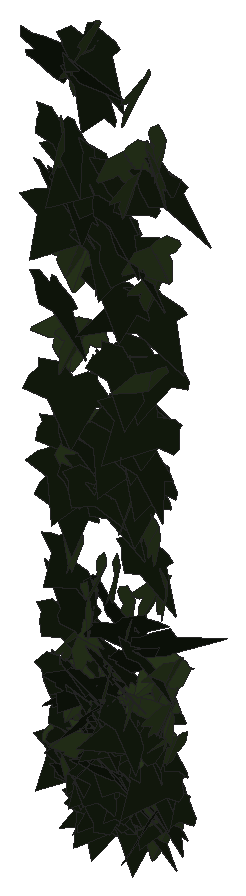
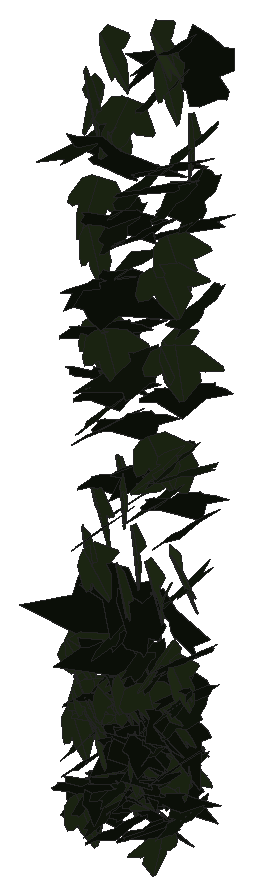
# SketchUp Ruby script. Lengths in inches.
U = 1.inch
M = Sketchup.active_model
def pt(a) = Geom::Point3d.new(a.map { |v| v * U })
def face(e, loops, mat)
  f = e.add_face(loops[0].map { |a| pt(a) })
  loops[1..].each { |l| e.add_face(l.map { |a| pt(a) }).erase! }
  f.material = f.back_material = mat if mat
  f
end
# faces: each face lists its corners as indices into pts; further lists are holes
def faces(e, pts, list, mat = nil) = list.each { |f| face(e, (f[0].is_a?(Array) ? f : [f]).map { |l| l.map { |i| pts[i] } }, mat) }
# xy, xz, yz: faces in a plane at the given z, y or x. An outline is a flat list of corners, or four numbers for a rectangle; further outlines are holes
def ring(l) = l.size == 4 ? [[l[0], l[1]], [l[2], l[1]], [l[2], l[3]], [l[0], l[3]]] : l.each_slice(2).to_a
def flat(e, list, mat, &to3) = list.each { |f| face(e, (f[0].is_a?(Array) ? f : [f]).map { |l| ring(l).map { |u, v| to3.(u, v) } }, mat) }
def xy(e, z, list, mat = nil) = flat(e, list, mat) { |x, y| [x, y, z] }
def xz(e, y, list, mat = nil) = flat(e, list, mat) { |x, z| [x, y, z] }
def yz(e, x, list, mat = nil) = flat(e, list, mat) { |y, z| [x, y, z] }
def lines(e, pts, list) = list.each { |a, b| e.add_line(pt(pts[a]), pt(pts[b])) }
# prism: a flat outline (further loops are holes) pulled along v
def prism(e, loops, v, mat = nil)
  f = face(e, loops, mat); d = Geom::Vector3d.new(v.map { |x| x * U })
  f.pushpull(f.normal.samedirection?(d) ? d.length : -d.length)
end
def box(e, o, s, mat = nil) = prism(e, [[o, [o[0] + s[0], o[1], o[2]], [o[0] + s[0], o[1] + s[1], o[2]], [o[0], o[1] + s[1], o[2]]]], [0, 0, s[2]], mat)
def at(x, y, z, deg = 0) = Geom::Transformation.translation(pt([x, y, z])) * Geom::Transformation.rotation(ORIGIN, Z_AXIS, deg.degrees)
def axes(o, x, y, z) = Geom::Transformation.new([*x, 0, *y, 0, *z, 0, *pt(o).to_a, 1])
def part(name) = M.definitions.add(name)
# library, detail: a bought-in or finely detailed component or shape, given as its bounding box
def library(name, o, s) = part(name).tap { |d| box(d.entities, o, s) }
def detail(e, o, s) = box(e.add_group.entities, o, s)
def put(e, d, t, mat = nil) = e.add_instance(d, t).tap { |i| i.material = mat if mat }
def group(e, t, mat = nil) = e.add_group.tap { |g| g.transformation = t; g.material = mat if mat }.entities
root = M.entities
M.materials.add("1026 AP 7946 SUNNY SIDE UP").color = [254, 231, 186]
M.materials.add("efeu1").color = [18, 25, 13]
M.materials.add("efeu2").color = [43, 57, 29]
c1 = part("ivyleaf_9")
p = [[1.54,2.16,1.25],[1.36,2.04,1.19],[-0.21,0.99,0.68],[-0.71,1.11,0.82],[-0.85,0.86,0.67],[-0.8,0.17,0.21],
  [-0.9,-0.01,0.1],[-0.67,-0.16,-0.02],[-0.08,-0.08,-0.05],[-0.03,-0.6,-0.4],[0.65,-0.88,-0.66],[0.83,-0.6,-0.49],
  [1.29,-0.42,-0.43],[1.8125,-0.07,-0.26],[1.21,0.44,0.15]]
faces(c1.entities,p,[[0,1,2,3,4,5,6,7,8,9,10,11,12,13,14]],"efeu1")
c2 = part("ivyleaf_10")
p = [[0,0.5,-0.03],[-0.0625,2.02,-0.43],[-0.19,2.01,-0.46],[-0.54,1.05,-0.29],[-0.52,0.625,-0.18],[-0.83,0.76,-0.28],
  [-1.16,0.64,-0.33],[-1.15,0.33,-0.24],[-0.77,-0.39,0.02],[-0.3,-0.51,0.16],[0.04,-0.48,0.23],[-0.02,2.01,-0.4375],
  [-0.06,2.01,-0.43],[0.04,-0.49,0.23],[0.67,-0.49,0.14],[1.38,0.36,-0.2],[1.375,0.51,-0.24],[0.81,0.65,-0.19],
  [0.62,0.59,-0.15],[0.6,1.09,-0.28],[0.5,1.23,-0.31]]
faces(c2.entities,p,[[0,1,2,3,4,5,6,7,8,9,10],[11,12,0,13,14,15,16,17,18,19,20]],"efeu2")
put(root,c1,axes([113.48,212.84,268.6],[-0.35522,-0.12905,0.0337],[-0.02324,-0.04117,-0.26669],[0.20833,-0.22463,0.02772]),"1026 AP 7946 SUNNY SIDE UP")
put(root,c2,axes([113.42,212.75,274.85],[-0.34565,-0.19628,0.04579],[0.03173,-0.08853,-0.29313],[0.31524,-0.2063,0.07971]),"1026 AP 7946 SUNNY SIDE UP")
put(root,c1,axes([113.22,212.86,268.37],[0.02902,-0.2292,0.12467],[0.0477,-0.11988,-0.23684],[0.40571,0.03049,0.01893]),"1026 AP 7946 SUNNY SIDE UP")
put(root,c1,axes([113.54,212.62,269.58],[-0.0128,0.25552,-0.08031],[-0.00758,-0.07957,-0.26373],[-0.42067,-0.00634,0.0072]),"1026 AP 7946 SUNNY SIDE UP")
put(root,c1,axes([113.16,212.56,277.08],[0.26409,-0.24942,0.06151],[0.02497,-0.0628,-0.30935],[0.40301,0.16733,-0.02114]),"1026 AP 7946 SUNNY SIDE UP")
put(root,c1,axes([113.01,212.5,278.9],[0.34286,-0.0936,0.22032],[0.2876,-0.11451,-0.24381],[0.22933,0.28355,-0.02363]),"1026 AP 7946 SUNNY SIDE UP")
put(root,c1,axes([113.46,212.61,276.61],[-0.26398,-0.218,0.1356],[-0.05261,-0.13886,-0.27908],[0.39797,-0.16296,0.05305]),"1026 AP 7946 SUNNY SIDE UP")
put(root,c1,axes([113.21,212.49,275.5],[0.19609,-0.27684,0.01941],[-0.00452,-0.02367,-0.31268],[0.43646,0.12413,-0.01196]),"1026 AP 7946 SUNNY SIDE UP")
put(root,c2,axes([113.47,212.67,270.32],[0.05534,-0.26982,0.04445],[0.00724,-0.04446,-0.28058],[0.42998,0.03548,-0.001]),"1026 AP 7946 SUNNY SIDE UP")
put(root,c1,axes([113.26,212.65,277.83],[0.08075,-0.29984,0.06282],[0.00263,-0.06328,-0.31363],[0.48166,0.05061,-0.00882]),"1026 AP 7946 SUNNY SIDE UP")
put(root,c1,axes([113.47,212.75,272.8125],[-0.26999,-0.22959,0.01881],[0.00256,-0.02561,-0.29501],[0.36231,-0.17091,0.0161]),"1026 AP 7946 SUNNY SIDE UP")
put(root,c1,axes([113.29,212.71,270.61],[0.05901,-0.26443,-0.07652],[0.03601,0.07622,-0.27269],[0.42975,0.02993,0.03336]),"1026 AP 7946 SUNNY SIDE UP")
put(root,c1,axes([113.35,212.71,272.41],[-0.03389,-0.28188,0.05813],[-0.00825,-0.05779,-0.29158],[0.45245,-0.02217,-0.00096]),"1026 AP 7946 SUNNY SIDE UP")
put(root,c1,axes([113.32,212.87,268.32],[0.08214,-0.25847,0.00442],[-0.01193,-0.0074,-0.27155],[0.40635,0.05203,-0.00886]),"1026 AP 7946 SUNNY SIDE UP")
put(root,c2,axes([113.35,212.77,269.06],[-0.25776,0.13858,-0.15599],[0.14481,-0.12463,-0.21982],[-0.28946,-0.18575,0.02893]),"1026 AP 7946 SUNNY SIDE UP")
put(root,c2,axes([113.53,212.86,276],[-0.28419,-0.21443,0.093],[0.0063,-0.1186,-0.27891],[0.36652,-0.16422,0.0769]),"1026 AP 7946 SUNNY SIDE UP")
put(root,c1,axes([113.32,212.83,269.125],[0.04833,-0.26355,-0.0045],[-0.00045,0.00286,-0.27333],[0.41443,0.03074,0.00023]),"1026 AP 7946 SUNNY SIDE UP")
put(root,c1,axes([113.46,212.66,271.42],[-0.1428,-0.14223,0.23774],[-0.06464,-0.23417,-0.16614],[0.42242,-0.08392,0.05495]),"1026 AP 7946 SUNNY SIDE UP")
put(root,c1,axes([113.75,212.4375,270.84],[-0.04211,0.06084,0.28221],[-0.19288,0.24457,-0.06697],[-0.39625,-0.12552,0.00261]),"1026 AP 7946 SUNNY SIDE UP")
put(root,c2,axes([113.57,212.63,276.29],[-0.12507,-0.29128,0.04301],[-0.00437,-0.04422,-0.31119],[0.46305,-0.07909,0.00868]),"1026 AP 7946 SUNNY SIDE UP")
put(root,c2,axes([113.52,212.3125,277.88],[0.16277,-0.27111,-0.13087],[0.02936,0.13842,-0.2914],[0.46884,0.08546,0.06368]),"1026 AP 7946 SUNNY SIDE UP")
put(root,c2,axes([113.55,212.8,278.88],[0.0131,-0.31323,-0.0052],[0.00308,0.00332,-0.32278],[0.49255,0.00831,0.00216]),"1026 AP 7946 SUNNY SIDE UP")
put(root,c1,axes([113.32,212.82,273.23],[-0.05087,-0.2826,0.02781],[0.15931,-0.03837,-0.27277],[0.41725,-0.0198,0.10754]),"1026 AP 7946 SUNNY SIDE UP")
put(root,c2,axes([113.54,212.56,271.76],[0.26992,-0.24753,0.01645],[-0.00644,-0.02396,-0.30997],[0.39013,0.17087,-0.01651]),"1026 AP 7946 SUNNY SIDE UP")
put(root,c2,axes([113.54,212.6875,274.89],[-0.00025,-0.25006,0.16976],[0.0574,-0.16499,-0.25665],[0.46862,0.02007,0.03153]),"1026 AP 7946 SUNNY SIDE UP")
put(root,c2,axes([113.55,212.68,269.63],[0.32708,-0.17486,-0.00281],[-0.02066,-0.01294,-0.27939],[0.27419,0.20762,-0.0177]),"1026 AP 7946 SUNNY SIDE UP")
put(root,c1,axes([113.37,212.8,269.66],[-0.04577,-0.19768,0.19034],[0.12471,-0.18499,-0.19095],[0.40804,0.03436,0.07971]),"1026 AP 7946 SUNNY SIDE UP")
put(root,c1,axes([113.375,212.54,270.01],[0.10974,-0.20238,-0.17601],[0.00466,0.17612,-0.21409],[0.41527,0.05151,0.04891]),"1026 AP 7946 SUNNY SIDE UP")
put(root,c2,axes([113.67,212.875,273.52],[-0.18295,-0.24391,0.0981],[-0.00097,-0.10543,-0.27559],[0.41251,-0.10842,0.04286]),"1026 AP 7946 SUNNY SIDE UP")
put(root,c1,axes([113.55,212.51,274.23],[-0.19164,-0.2676,-0.05532],[0.05157,0.04235,-0.30243],[0.42559,-0.12563,0.01174]),"1026 AP 7946 SUNNY SIDE UP")
put(root,c2,axes([113.63,212.8,279.27],[0.16707,-0.26335,0.1327],[0.04344,-0.129,-0.29253],[0.45996,0.10784,-0.02057]),"1026 AP 7946 SUNNY SIDE UP")
put(root,c1,axes([113.43,212.76,273.35],[0.15787,-0.27032,0.01008],[0.02044,-0.00724,-0.29694],[0.42493,0.10077,0.01054]),"1026 AP 7946 SUNNY SIDE UP")
put(root,c2,axes([113.49,212.58,273.26],[-0.02297,-0.16286,-0.29283],[0.26291,0.23995,-0.14957],[0.44151,-0.15136,0.07383]),"1026 AP 7946 SUNNY SIDE UP")
put(root,c2,axes([113.54,212.61,268.96],[0.43626,0.02874,0.04187],[0.06746,-0.02319,-0.28612],[-0.03927,0.27942,-0.02639]),"1026 AP 7946 SUNNY SIDE UP")
put(root,c1,axes([113.69,212.8,268.77],[-0.23684,-0.21018,0.04816],[-0.01429,-0.05224,-0.26566],[0.33867,-0.14918,0.02247]),"1026 AP 7946 SUNNY SIDE UP")
put(root,c2,axes([113.83,212.76,268.85],[-0.21979,-0.13195,0.18222],[-0.11105,-0.17251,-0.19028],[0.32974,-0.14605,0.05738]),"1026 AP 7946 SUNNY SIDE UP")
put(root,c1,axes([113.74,212.6875,277.39],[-0.29422,-0.1988,0.13242],[-0.04731,-0.14391,-0.27288],[0.3702,-0.17639,0.07037]),"1026 AP 7946 SUNNY SIDE UP")
put(root,c1,axes([113.53,212.625,276.97],[0.01826,-0.24914,0.18214],[0.02229,-0.17772,-0.25793],[0.48114,0.01769,0.00504]),"1026 AP 7946 SUNNY SIDE UP")
put(root,c1,axes([113.52,212.5,269.99],[0.33229,-0.15585,-0.07552],[-0.07407,0.05787,-0.26954],[0.25988,0.21577,0.01975]),"1026 AP 7946 SUNNY SIDE UP")
put(root,c2,axes([113.79,212.45,268.99],[-0.13395,-0.24571,0.08396],[-0.01971,-0.08324,-0.26797],[0.40727,-0.08484,0.01464]),"1026 AP 7946 SUNNY SIDE UP")
put(root,c1,axes([113.55,212.78,279.15],[0.1266,-0.28099,-0.12066],[-0.03861,0.11311,-0.30038],[0.47616,0.08388,0.00772]),"1026 AP 7946 SUNNY SIDE UP")
put(root,c1,axes([113.57,212.58,268.77],[-0.04031,-0.23664,0.12685],[0.07487,-0.12709,-0.23955],[0.41372,-0.00006,0.05571]),"1026 AP 7946 SUNNY SIDE UP")
put(root,c1,axes([113.56,212.73,269.77],[0.12371,-0.26151,0.00051],[0.00778,-0.00058,-0.2813],[0.41114,0.0787,0.00517]),"1026 AP 7946 SUNNY SIDE UP")
put(root,c1,axes([113.5625,212.55,272.875],[0.26404,-0.18707,-0.14183],[-0.07107,0.13902,-0.25255],[0.35724,0.16593,0.05458]),"1026 AP 7946 SUNNY SIDE UP")
put(root,c2,axes([113.8125,212.81,269.96],[-0.29711,-0.18819,0.06439],[0.01664,-0.09715,-0.26444],[0.31189,-0.17409,0.07544]),"1026 AP 7946 SUNNY SIDE UP")
put(root,c2,axes([113.72,212.71,267.83],[0.11179,0.24781,-0.00301],[-0.01534,-0.0017,-0.26545],[-0.38942,0.07121,0.00959]),"1026 AP 7946 SUNNY SIDE UP")
put(root,c1,axes([113.86,212.61,269.38],[-0.21473,0.06497,-0.22243],[0.14834,-0.21322,-0.1286],[-0.32262,-0.14128,0.08892]),"1026 AP 7946 SUNNY SIDE UP")
put(root,c1,axes([113.78,212.95,277.2],[-0.26953,-0.22433,0.0929],[-0.00009,-0.11199,-0.28378],[0.38092,-0.15876,0.06567]),"1026 AP 7946 SUNNY SIDE UP")
put(root,c1,axes([113.68,212.79,278.48],[-0.06963,-0.22261,0.21034],[-0.00907,-0.20696,-0.23353],[0.47623,-0.03649,0.0263]),"1026 AP 7946 SUNNY SIDE UP")
put(root,c2,axes([113.72,212.5,270.44],[0.06807,-0.20259,-0.22166],[0.16254,0.213,-0.18494],[0.43394,-0.04801,0.10404]),"1026 AP 7946 SUNNY SIDE UP")
put(root,c1,axes([113.95,212.35,270],[0.15929,0.17617,-0.20067],[-0.17144,-0.1629,-0.21008],[-0.37699,0.14852,0.01075]),"1026 AP 7946 SUNNY SIDE UP")
put(root,c1,axes([113.88,212.86,269.33],[-0.12185,0.11527,-0.23404],[0.1547,-0.20623,-0.14317],[-0.37049,-0.12402,0.01719]),"1026 AP 7946 SUNNY SIDE UP")
put(root,c1,axes([113.93,212.42,268.73],[-0.13152,0.18945,-0.20725],[-0.15819,0.1761,0.21381],[0.40602,0.12997,0.01617]),"1026 AP 7946 SUNNY SIDE UP")
put(root,c1,axes([113.91,212.74,267.95],[-0.19676,-0.19953,0.11969],[-0.04433,-0.11923,-0.24059],[0.36124,-0.12331,0.03567]),"1026 AP 7946 SUNNY SIDE UP")
put(root,c2,axes([113.95,212.58,271.51],[0.1304,-0.26022,-0.06907],[-0.03004,0.06272,-0.28099],[0.42089,0.0851,0.00134]),"1026 AP 7946 SUNNY SIDE UP")
put(root,c1,axes([113.69,212.375,268.59],[0.40539,0.06891,0.05745],[0.09123,-0.00307,-0.27434],[-0.10488,0.26368,-0.01656]),"1026 AP 7946 SUNNY SIDE UP")
put(root,c2,axes([113.79,212.63,271.01],[-0.00705,-0.09819,0.27508],[0.24705,-0.22413,-0.08333],[0.37393,0.14623,0.06024]),"1026 AP 7946 SUNNY SIDE UP")
put(root,c1,axes([114.07,212.85,269.23],[-0.38875,-0.10692,0.00549],[0.00653,-0.02451,-0.27652],[0.16825,-0.24609,0.02343]),"1026 AP 7946 SUNNY SIDE UP")
put(root,c2,axes([113.95,212.86,268.91],[0.03549,-0.23859,0.11226],[0.05779,-0.10678,-0.24627],[0.40927,0.03577,0.02504]),"1026 AP 7946 SUNNY SIDE UP")
put(root,c1,axes([113.93,212.73,267.97],[-0.14196,-0.23832,0.04227],[-0.01906,-0.04073,-0.26276],[0.38014,-0.09104,0.00261]),"1026 AP 7946 SUNNY SIDE UP")
put(root,c1,axes([114.33,212.68,269.55],[-0.18353,-0.01532,-0.27288],[-0.41612,-0.01263,0.12085],[-0.0279,0.2891,-0.00748]),"1026 AP 7946 SUNNY SIDE UP")
put(root,c1,axes([113.8,212.86,269.1],[0.02233,-0.22202,0.14867],[0.07158,-0.14159,-0.22786],[0.41127,0.0367,0.03159]),"1026 AP 7946 SUNNY SIDE UP")
put(root,c1,axes([114.11,212.57,269.05],[0.02433,0.26408,-0.04313],[-0.00187,-0.04336,-0.27277],[-0.4208,0.01546,-0.00128]),"1026 AP 7946 SUNNY SIDE UP")
put(root,c1,axes([114.23,212.65,268.1875],[-0.40647,0.02011,0.01816],[-0.03031,-0.02295,-0.26607],[-0.02897,-0.25808,0.02355]),"1026 AP 7946 SUNNY SIDE UP")
put(root,c1,axes([113.78,212.89,270.84],[0.08297,-0.10308,0.27017],[0.16315,-0.2416,-0.12048],[0.41287,0.11618,-0.00669]),"1026 AP 7946 SUNNY SIDE UP")
put(root,c1,axes([114.14,212.6,268.7],[-0.30564,-0.16748,0.05907],[-0.04938,-0.05261,-0.26392],[0.27444,-0.19599,0.0183]),"1026 AP 7946 SUNNY SIDE UP")
put(root,c1,axes([113.9,212.5625,270.25],[0.34195,-0.1571,-0.05565],[-0.05527,0.04195,-0.2758],[0.25484,0.2199,0.01485]),"1026 AP 7946 SUNNY SIDE UP")
put(root,c2,axes([114.17,212.82,269.95],[-0.02456,-0.26346,0.06621],[-0.01442,-0.06533,-0.27223],[0.42674,-0.01737,-0.00539]),"1026 AP 7946 SUNNY SIDE UP")
put(root,c1,axes([114.07,212.71,276.35],[-0.13488,-0.26769,0.09834],[-0.00744,-0.09993,-0.28906],[0.44763,-0.08232,0.02483]),"1026 AP 7946 SUNNY SIDE UP")
put(root,c1,axes([113.98,212.39,268.61],[0.16248,-0.21725,-0.13266],[-0.03045,0.13059,-0.24457],[0.39495,0.09945,0.03572]),"1026 AP 7946 SUNNY SIDE UP")
put(root,c1,axes([113.98,212.49,272.97],[0.02788,-0.2325,-0.17727],[0.05557,0.17154,-0.23584],[0.45017,-0.00677,0.04009]),"1026 AP 7946 SUNNY SIDE UP")
put(root,c1,axes([114,212.6,269.15],[0.36101,0.11379,0.059],[0.08437,0.01921,-0.26378],[-0.18117,0.23569,-0.00528]),"1026 AP 7946 SUNNY SIDE UP")
put(root,c1,axes([114.27,212.81,269.21],[-0.26195,-0.16712,0.13489],[-0.12476,-0.10665,-0.24311],[0.31063,-0.18377,0.0161]),"1026 AP 7946 SUNNY SIDE UP")
put(root,c2,axes([114.21,212.41,270.17],[0.16755,-0.23559,-0.08579],[0.00138,0.08946,-0.26327],[0.39221,0.10033,0.03758]),"1026 AP 7946 SUNNY SIDE UP")
put(root,c1,axes([114,212.67,272.67],[0.13522,-0.27164,-0.06144],[0.00499,0.06177,-0.29236],[0.43677,0.08339,0.02236]),"1026 AP 7946 SUNNY SIDE UP")
put(root,c1,axes([114.35,212.52,268.36],[-0.38517,0.05437,-0.07268],[0.09322,-0.05575,-0.25551],[-0.10505,-0.24883,0.03977]),"1026 AP 7946 SUNNY SIDE UP")
put(root,c1,axes([114.39,212.55,269.9],[-0.18631,0.22856,-0.09657],[0.03495,-0.09512,-0.26476],[-0.38765,-0.11843,0.02254]),"1026 AP 7946 SUNNY SIDE UP")
put(root,c1,axes([113.94,212.74,274.49],[0.37848,-0.17443,-0.02157],[0.03093,0.06043,-0.29951],[0.27433,0.23384,0.06353]),"1026 AP 7946 SUNNY SIDE UP")
put(root,c1,axes([114.34,212.88,268.61],[-0.33443,-0.13962,0.07289],[-0.04695,-0.0823,-0.25738],[0.24217,-0.20876,0.05076]),"1026 AP 7946 SUNNY SIDE UP")
put(root,c1,axes([114.08,212.58,270.34],[0.35123,-0.1227,-0.10434],[-0.09749,0.09237,-0.2574],[0.22964,0.22689,0.0503]),"1026 AP 7946 SUNNY SIDE UP")
put(root,c1,axes([114.33,212.45,268],[-0.22003,-0.1383,0.20503],[0.19253,0.15903,0.20267],[-0.33005,0.18497,-0.01846]),"1026 AP 7946 SUNNY SIDE UP")
put(root,c1,axes([114.46,212.89,275.51],[-0.06682,0.02081,-0.29913],[0.0056,-0.2935,-0.02392],[-0.4579,-0.00663,0.04336]),"1026 AP 7946 SUNNY SIDE UP")
put(root,c1,axes([114.1,212.67,276.91],[0.12897,-0.28858,0.0636],[0.01331,-0.06345,-0.3093],[0.46438,0.08196,-0.0088]),"1026 AP 7946 SUNNY SIDE UP")
put(root,c1,axes([114.69,212.72,277.27],[-0.19234,0.10061,0.26426],[-0.40026,0.06457,-0.15111],[-0.16362,-0.27622,0.05901]),"1026 AP 7946 SUNNY SIDE UP")
put(root,c2,axes([114.41,212.55,269.67],[0.1692,-0.21465,-0.13524],[-0.08491,0.11839,-0.24663],[0.3854,0.12032,0.00504]),"1026 AP 7946 SUNNY SIDE UP")
put(root,c2,axes([114.62,212.62,268.35],[0.05817,0.03009,-0.28061],[-0.37742,0.13654,-0.01724],[0.20849,0.23878,0.04709]),"1026 AP 7946 SUNNY SIDE UP")
put(root,c1,axes([114.35,212.62,273.58],[-0.26744,-0.23386,0.02219],[-0.01144,-0.02298,-0.29793],[0.3693,-0.17007,0.00684]),"1026 AP 7946 SUNNY SIDE UP")
put(root,c1,axes([114.43,212.76,276.51],[-0.35983,-0.19465,0.01969],[-0.00148,-0.03001,-0.30883],[0.30772,-0.22777,0.02153]),"1026 AP 7946 SUNNY SIDE UP")
put(root,c1,axes([114.22,212.61,275.82],[-0.0586,-0.27084,0.13304],[0.05018,-0.1345,-0.27858],[0.47018,-0.0194,0.04631]),"1026 AP 7946 SUNNY SIDE UP")
put(root,c2,axes([114.4,212.34,271.74],[0.14434,-0.25696,-0.09129],[0.00835,0.09369,-0.27826],[0.42658,0.08511,0.03634]),"1026 AP 7946 SUNNY SIDE UP")
put(root,c1,axes([114.09,212.58,268.56],[0.2937,-0.17455,0.12171],[0.11364,-0.09665,-0.26318],[0.31226,0.19935,-0.0187]),"1026 AP 7946 SUNNY SIDE UP")
put(root,c2,axes([114.46,212.54,272.79],[0.15423,-0.26079,-0.17883],[-0.04143,0.17284,-0.28427],[0.48957,0.09679,0.03228]),"1026 AP 7946 SUNNY SIDE UP")
put(root,c1,axes([114.3125,212.85,267.89],[-0.07657,-0.25585,0.03477],[-0.00323,-0.03544,-0.26847],[0.40608,-0.04852,0.00442]),"1026 AP 7946 SUNNY SIDE UP")
put(root,c2,axes([114.48,212.53,268.52],[0.25413,-0.19926,-0.08662],[-0.07195,0.06964,-0.26378],[0.33167,0.16779,0.00915]),"1026 AP 7946 SUNNY SIDE UP")
put(root,c2,axes([114.52,212.75,274.7],[-0.20511,-0.25863,0.03839],[-0.00753,-0.04091,-0.2983],[0.41114,-0.12977,0.01369]),"1026 AP 7946 SUNNY SIDE UP")
put(root,c2,axes([114.5,212.49,271.22],[0.21985,-0.22938,-0.12012],[-0.04457,0.1167,-0.27389],[0.40121,0.13866,0.0354]),"1026 AP 7946 SUNNY SIDE UP")
put(root,c1,axes([114.38,212.8,272.88],[-0.11988,-0.27444,-0.00786],[0.01068,0.00442,-0.29336],[0.43151,-0.07636,0.00508]),"1026 AP 7946 SUNNY SIDE UP")
put(root,c2,axes([114.5625,212.65,269.71],[-0.36966,-0.11472,0.04379],[-0.04477,-0.03968,-0.26869],[0.18746,-0.23571,0.02218]),"1026 AP 7946 SUNNY SIDE UP")
put(root,c1,axes([114.26,212.78,268.54],[0.2371,-0.21399,0.0016],[0.00559,-0.00089,-0.26968],[0.33646,0.15081,0.00335]),"1026 AP 7946 SUNNY SIDE UP")
put(root,c2,axes([114.46,212.86,269.76],[-0.06048,-0.20314,0.17627],[0.08501,-0.17637,-0.20287],[0.41008,0.0066,0.06805]),"1026 AP 7946 SUNNY SIDE UP")
put(root,c1,axes([114.47,212.28,271.03],[0.25003,0.23531,-0.01828],[0.00187,-0.0238,-0.29234],[-0.37121,0.15837,-0.01379]),"1026 AP 7946 SUNNY SIDE UP")
put(root,c1,axes([114.25,212.72,276.41],[0.21604,-0.25444,0.07224],[0.04342,-0.0664,-0.2982],[0.41333,0.13997,-0.00643]),"1026 AP 7946 SUNNY SIDE UP")
put(root,c2,axes([114.53,212.82,269.04],[0.09247,-0.25911,0.03744],[0.00869,-0.03752,-0.27392],[0.41164,0.05899,-0.00263]),"1026 AP 7946 SUNNY SIDE UP")
put(root,c2,axes([114.54,212.69,278.86],[0.11025,-0.29827,0.05834],[0.00457,-0.0592,-0.31581],[0.47786,0.06938,-0.01044]),"1026 AP 7946 SUNNY SIDE UP")
put(root,c2,axes([114.47,212.47,277.86],[-0.17134,-0.24381,-0.1661],[0.13451,0.1364,-0.27361],[0.43824,-0.13719,0.01904]),"1026 AP 7946 SUNNY SIDE UP")
put(root,c1,axes([114.29,212.58,270.28],[0.2817,0.09777,0.18782],[0.23984,0.09941,-0.20939],[-0.2186,0.23505,0.0123]),"1026 AP 7946 SUNNY SIDE UP")
put(root,c1,axes([114.72,212.61,269.39],[-0.33067,-0.08373,0.1533],[-0.17938,-0.10772,-0.22844],[0.20064,-0.23432,0.04841]),"1026 AP 7946 SUNNY SIDE UP")
put(root,c1,axes([114.42,212.56,269.58],[0.00454,-0.26167,0.03561],[0.00027,-0.03606,-0.2698],[0.41534,0.00288,-0.00022]),"1026 AP 7946 SUNNY SIDE UP")
put(root,c1,axes([114.49,212.53,274.77],[-0.13092,-0.27875,0.01226],[0.00707,-0.01541,-0.29966],[0.43876,-0.08293,0.00849]),"1026 AP 7946 SUNNY SIDE UP")
put(root,c2,axes([114.5,212.66,269.41],[0.27584,0.20496,-0.0112],[0.01055,-0.02154,-0.27736],[-0.32267,0.17451,-0.01864]),"1026 AP 7946 SUNNY SIDE UP")
put(root,c1,axes([114.37,212.73,270.58],[0.21022,-0.24238,0.01165],[0.02112,-0.00707,-0.28508],[0.38106,0.13411,0.00937]),"1026 AP 7946 SUNNY SIDE UP")
put(root,c2,axes([114.64,212.41,277.6],[0.04311,-0.30689,-0.02054],[0.00745,0.01868,-0.31724],[0.48335,0.02709,0.00672]),"1026 AP 7946 SUNNY SIDE UP")
put(root,c2,axes([114.67,212.79,269.7],[-0.28028,-0.19981,0.04544],[0.01368,-0.0673,-0.27128],[0.32185,-0.17115,0.0511]),"1026 AP 7946 SUNNY SIDE UP")
put(root,c1,axes([114.5625,212.64,273.97],[-0.18416,-0.26749,-0.01228],[0.01655,0.00675,-0.3007],[0.4206,-0.11739,0.00645]),"1026 AP 7946 SUNNY SIDE UP")
put(root,c1,axes([114.43,212.84,268.07],[0.18095,-0.23777,0.01113],[0.01011,-0.01039,-0.27219],[0.37422,0.11525,0.00198]),"1026 AP 7946 SUNNY SIDE UP")
put(root,c1,axes([114.56,212.8,269.67],[-0.09722,-0.25096,-0.08238],[0.04921,0.07309,-0.26553],[0.41054,-0.06819,0.01232]),"1026 AP 7946 SUNNY SIDE UP")
put(root,c1,axes([114.49,212.8,275.56],[0.01781,-0.26699,-0.14101],[0.08131,0.13517,-0.2694],[0.4636,-0.01345,0.05267]),"1026 AP 7946 SUNNY SIDE UP")
put(root,c2,axes([114.75,212.74,276.07],[-0.03803,-0.29391,-0.00856],[0.00497,0.00641,-0.30376],[0.46224,-0.02425,0.00256]),"1026 AP 7946 SUNNY SIDE UP")
put(root,c1,axes([114.67,212.76,274.84],[-0.24004,-0.2554,-0.01765],[0.03894,0.00342,-0.30585],[0.40046,-0.15342,0.01917]),"1026 AP 7946 SUNNY SIDE UP")
put(root,c2,axes([114.78,212.62,272.36],[0.25681,-0.19757,-0.12503],[-0.06918,0.11797,-0.26057],[0.35703,0.16497,0.03944]),"1026 AP 7946 SUNNY SIDE UP")
put(root,c2,axes([114.76,212.77,271.5],[-0.01006,-0.26429,0.08873],[0.00737,-0.08774,-0.27278],[0.43775,-0.0046,0.00663]),"1026 AP 7946 SUNNY SIDE UP")
put(root,c1,axes([114.84,212.58,274.08],[-0.40052,-0.13995,0.02943],[0.0012,-0.06132,-0.29458],[0.22484,-0.24896,0.05401]),"1026 AP 7946 SUNNY SIDE UP")
put(root,c1,axes([114.79,212.69,268.17],[-0.19513,0.11414,-0.21025],[0.20289,-0.16014,-0.17348],[-0.30771,-0.17797,0.01894]),"1026 AP 7946 SUNNY SIDE UP")
put(root,c2,axes([114.86,212.9,270.3],[-0.19504,-0.13207,0.20687],[-0.05953,-0.2132,-0.16916],[0.3742,-0.10275,0.08092]),"1026 AP 7946 SUNNY SIDE UP")
put(root,c1,axes([114.58,212.66,272.03],[0.12547,-0.26339,-0.0627],[-0.00834,0.06036,-0.28289],[0.42446,0.07904,0.01297]),"1026 AP 7946 SUNNY SIDE UP")
put(root,c1,axes([114.77,212.9,268.34],[-0.2962,-0.18136,-0.01693],[0.06886,-0.02365,-0.26507],[0.27779,-0.18752,0.04766]),"1026 AP 7946 SUNNY SIDE UP")
put(root,c2,axes([114.8125,212.5,274.68],[-0.15229,-0.28507,-0.01581],[0.02582,0.00891,-0.30984],[0.44803,-0.09741,0.01248]),"1026 AP 7946 SUNNY SIDE UP")
put(root,c1,axes([114.71,212.64,273.33],[-0.12033,-0.2598,0.11643],[-0.00651,-0.11754,-0.27832],[0.44638,-0.07175,0.02733]),"1026 AP 7946 SUNNY SIDE UP")
put(root,c2,axes([114.89,212.79,267.98],[-0.11641,-0.24521,0.05786],[-0.00555,-0.05898,-0.26386],[0.39601,-0.07291,0.01331]),"1026 AP 7946 SUNNY SIDE UP")
put(root,c2,axes([114.875,212.79,269.66],[0.01222,-0.26507,0.05481],[0.00609,-0.05462,-0.2735],[0.42553,0.0084,0.00234]),"1026 AP 7946 SUNNY SIDE UP")
put(root,c1,axes([114.71,212.82,268.75],[0.01575,-0.26466,0.02186],[0.00008,-0.02274,-0.27298],[0.41768,0.00999,-0.00077]),"1026 AP 7946 SUNNY SIDE UP")
put(root,c2,axes([114.93,212.58,278.125],[0.22959,-0.25634,-0.10766],[-0.03339,0.1058,-0.3015],[0.43313,0.14403,0.03383]),"1026 AP 7946 SUNNY SIDE UP")
put(root,c2,axes([114.94,212.79,270.32],[-0.03877,-0.26657,0.03706],[-0.0035,-0.03744,-0.276],[0.42326,-0.02473,0.00111]),"1026 AP 7946 SUNNY SIDE UP")
put(root,c1,axes([114.75,212.88,269.01],[0.04059,-0.25466,0.07496],[-0.0024,-0.0747,-0.26397],[0.41707,0.02436,-0.00882]),"1026 AP 7946 SUNNY SIDE UP")
put(root,c1,axes([114.73,212.52,273.52],[0.07287,-0.2793,0.04105],[0.00184,-0.04179,-0.29185],[0.44397,0.04601,-0.00553]),"1026 AP 7946 SUNNY SIDE UP")
put(root,c1,axes([114.98,212.57,268.88],[-0.38654,-0.06487,-0.07108],[0.13512,-0.07428,-0.2452],[0.06159,-0.24418,0.09181]),"1026 AP 7946 SUNNY SIDE UP")
put(root,c2,axes([114.9,212.48,277.96],[-0.25301,0.25653,-0.01267],[-0.00463,-0.01807,-0.31182],[-0.40392,-0.16048,0.01151]),"1026 AP 7946 SUNNY SIDE UP")
put(root,c2,axes([114.9,212.49,276.6],[-0.16992,-0.25737,-0.13334],[0.10858,0.10946,-0.28623],[0.43871,-0.12678,0.0192]),"1026 AP 7946 SUNNY SIDE UP")
put(root,c2,axes([114.97,212.82,269.22],[-0.04922,-0.26711,0.02505],[0.00129,-0.0261,-0.27718],[0.42196,-0.03107,0.00377]),"1026 AP 7946 SUNNY SIDE UP")
put(root,c2,axes([114.9,212.75,269.54],[0.28656,-0.1898,0.04524],[0.05048,-0.03154,-0.27125],[0.30253,0.18505,0.00241]),"1026 AP 7946 SUNNY SIDE UP")
put(root,c2,axes([114.93,212.83,269.86],[0.19994,-0.23518,0.04414],[0.03764,-0.03728,-0.27562],[0.37438,0.12935,0.00414]),"1026 AP 7946 SUNNY SIDE UP")
put(root,c1,axes([114.69,212.79,277.5],[0.23285,-0.26394,-0.05755],[0.04109,0.0758,-0.30536],[0.42173,0.13834,0.06153]),"1026 AP 7946 SUNNY SIDE UP")
put(root,c2,axes([114.99,212.57,271.63],[0.21994,-0.21749,-0.11367],[-0.02259,0.11824,-0.26111],[0.38194,0.13224,0.05001]),"1026 AP 7946 SUNNY SIDE UP")
put(root,c1,axes([114.75,212.85,268.13],[0.05156,-0.20422,0.15991],[0.10345,-0.14575,-0.21114],[0.391,0.06549,0.03478]),"1026 AP 7946 SUNNY SIDE UP")
put(root,c1,axes([114.71,212.61,270.625],[0.21037,0.01483,0.24769],[0.33634,0.11896,-0.12953],[-0.1739,0.24802,0.04911]),"1026 AP 7946 SUNNY SIDE UP")
